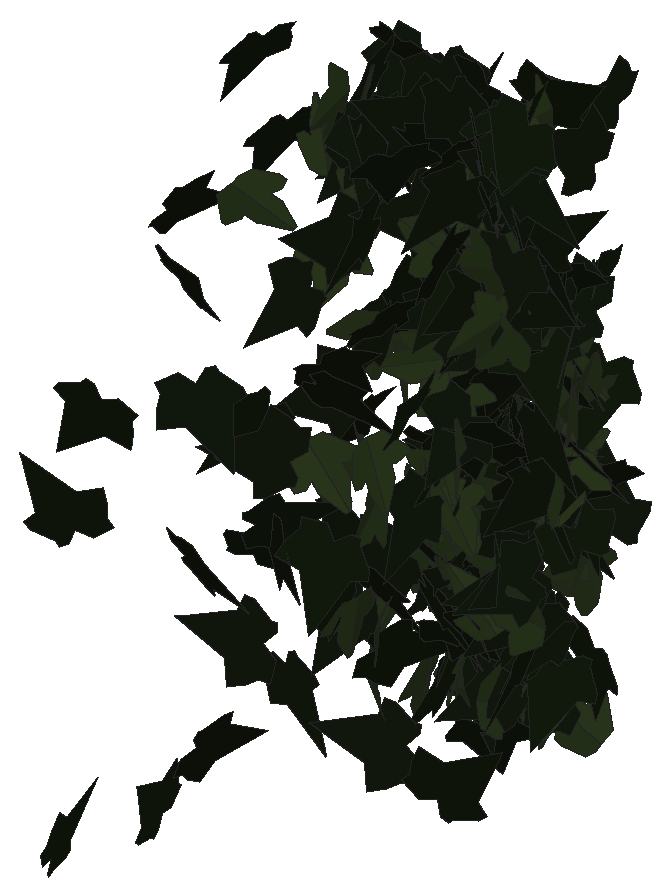
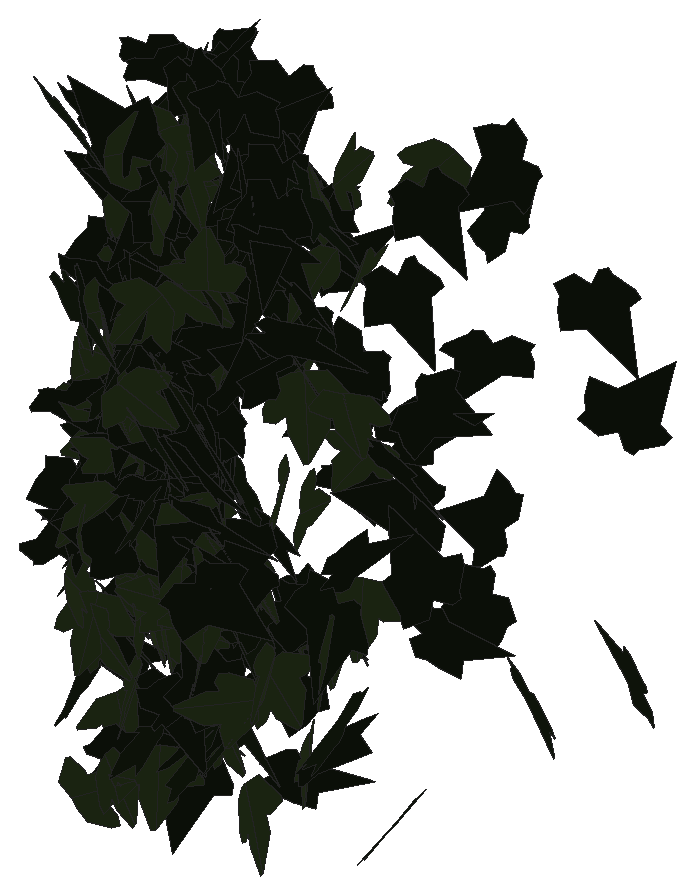
# SketchUp Ruby script. Lengths in inches.
U = 1.inch
M = Sketchup.active_model
def pt(a) = Geom::Point3d.new(a.map { |v| v * U })
def face(e, loops, mat)
  f = e.add_face(loops[0].map { |a| pt(a) })
  loops[1..].each { |l| e.add_face(l.map { |a| pt(a) }).erase! }
  f.material = f.back_material = mat if mat
  f
end
# faces: each face lists its corners as indices into pts; further lists are holes
def faces(e, pts, list, mat = nil) = list.each { |f| face(e, (f[0].is_a?(Array) ? f : [f]).map { |l| l.map { |i| pts[i] } }, mat) }
# xy, xz, yz: faces in a plane at the given z, y or x. An outline is a flat list of corners, or four numbers for a rectangle; further outlines are holes
def ring(l) = l.size == 4 ? [[l[0], l[1]], [l[2], l[1]], [l[2], l[3]], [l[0], l[3]]] : l.each_slice(2).to_a
def flat(e, list, mat, &to3) = list.each { |f| face(e, (f[0].is_a?(Array) ? f : [f]).map { |l| ring(l).map { |u, v| to3.(u, v) } }, mat) }
def xy(e, z, list, mat = nil) = flat(e, list, mat) { |x, y| [x, y, z] }
def xz(e, y, list, mat = nil) = flat(e, list, mat) { |x, z| [x, y, z] }
def yz(e, x, list, mat = nil) = flat(e, list, mat) { |y, z| [x, y, z] }
def lines(e, pts, list) = list.each { |a, b| e.add_line(pt(pts[a]), pt(pts[b])) }
# prism: a flat outline (further loops are holes) pulled along v
def prism(e, loops, v, mat = nil)
  f = face(e, loops, mat); d = Geom::Vector3d.new(v.map { |x| x * U })
  f.pushpull(f.normal.samedirection?(d) ? d.length : -d.length)
end
def box(e, o, s, mat = nil) = prism(e, [[o, [o[0] + s[0], o[1], o[2]], [o[0] + s[0], o[1] + s[1], o[2]], [o[0], o[1] + s[1], o[2]]]], [0, 0, s[2]], mat)
def at(x, y, z, deg = 0) = Geom::Transformation.translation(pt([x, y, z])) * Geom::Transformation.rotation(ORIGIN, Z_AXIS, deg.degrees)
def axes(o, x, y, z) = Geom::Transformation.new([*x, 0, *y, 0, *z, 0, *pt(o).to_a, 1])
def part(name) = M.definitions.add(name)
# library, detail: a bought-in or finely detailed component or shape, given as its bounding box
def library(name, o, s) = part(name).tap { |d| box(d.entities, o, s) }
def detail(e, o, s) = box(e.add_group.entities, o, s)
def put(e, d, t, mat = nil) = e.add_instance(d, t).tap { |i| i.material = mat if mat }
def group(e, t, mat = nil) = e.add_group.tap { |g| g.transformation = t; g.material = mat if mat }.entities
root = M.entities
M.materials.add("efeu1").color = [18, 25, 13]
M.materials.add("efeu2").color = [43, 57, 29]
c1 = part("ivyleaf_9")
p = [[1.54,2.16,1.25],[1.36,2.04,1.19],[-0.21,0.99,0.68],[-0.71,1.11,0.82],[-0.85,0.86,0.67],[-0.8,0.17,0.21],
  [-0.9,-0.01,0.1],[-0.67,-0.16,-0.02],[-0.08,-0.08,-0.05],[-0.03,-0.6,-0.4],[0.65,-0.88,-0.66],[0.83,-0.6,-0.49],
  [1.29,-0.42,-0.43],[1.8125,-0.07,-0.26],[1.21,0.44,0.15]]
faces(c1.entities,p,[[0,1,2,3,4,5,6,7,8,9,10,11,12,13,14]],"efeu1")
c2 = part("ivyleaf_10")
p = [[0,0.5,-0.03],[-0.0625,2.02,-0.43],[-0.19,2.01,-0.46],[-0.54,1.05,-0.29],[-0.52,0.625,-0.18],[-0.83,0.76,-0.28],
  [-1.16,0.64,-0.33],[-1.15,0.33,-0.24],[-0.77,-0.39,0.02],[-0.3,-0.51,0.16],[0.04,-0.48,0.23],[-0.02,2.01,-0.4375],
  [-0.06,2.01,-0.43],[0.04,-0.49,0.23],[0.67,-0.49,0.14],[1.38,0.36,-0.2],[1.375,0.51,-0.24],[0.81,0.65,-0.19],
  [0.62,0.59,-0.15],[0.6,1.09,-0.28],[0.5,1.23,-0.31]]
faces(c2.entities,p,[[0,1,2,3,4,5,6,7,8,9,10],[11,12,0,13,14,15,16,17,18,19,20]],"efeu2")
put(root,c1,axes([1.99,221.875,233.01],[-0.08667,0.34716,-0.25952],[0.03326,-0.24854,-0.3699],[-0.46054,-0.08328,0.02212]))
put(root,c1,axes([2.25,217.34,227.28],[0.20466,0.0164,0.40686],[-0.41836,0.07126,0.19203],[-0.06169,-0.42881,0.04747]))
put(root,c1,axes([2.25,222.11,231.66],[-0.04904,0.3605,-0.24874],[0.02338,-0.23829,-0.37781],[-0.46665,-0.04982,0.00721]))
put(root,c1,axes([2.48,222.28,229.01],[-0.46717,0.04349,-0.01539],[0.01585,-0.002,-0.45214],[-0.04701,-0.43282,0.00054]))
put(root,c1,axes([2.625,217.46,229.35],[0.16446,0.14018,-0.39791],[-0.29716,-0.26589,-0.21521],[-0.32459,0.31445,-0.00459]))
put(root,c2,axes([2.54,223.28,226.6],[-0.27724,0.37419,0.18198],[-0.15029,0.11386,-0.46309],[-0.38801,-0.31147,0.04934]))
put(root,c1,axes([2.81,222.76,227.24],[-0.16683,-0.15113,0.39263],[-0.24702,-0.30162,-0.2229],[0.36313,-0.27461,0.02875]))
put(root,c1,axes([2.79,222.78,226.72],[0.04672,0.47615,0.14526],[0.02368,0.14361,-0.47835],[-0.49725,0.05157,-0.00913]))
put(root,c1,axes([2.49,221.82,223.11],[0.22349,-0.37596,-0.07396],[-0.01378,0.07402,-0.44561],[0.41301,0.20591,0.02515]))
put(root,c1,axes([2.5,223,225.0625],[0.3031,-0.39745,-0.01273],[-0.00731,0.01043,-0.49984],[0.39759,0.30319,0.00051]))
put(root,c1,axes([2.71,216.32,222.62],[-0.16132,0.38355,0.14635],[0.04529,-0.13465,0.42797],[0.4389,0.15487,0.00963]))
put(root,c2,axes([2.93,222.1,226.56],[-0.45699,-0.09118,0.04487],[-0.04877,0.00485,-0.44993],[0.09742,-0.42531,-0.01475]))
put(root,c2,axes([2.8,222.51,229.72],[0.45214,0.11105,-0.0419],[-0.03967,-0.01863,-0.45037],[-0.12126,0.42017,-0.0089]))
put(root,c1,axes([2.77,218.87,231.89],[0.18453,0.28347,0.29356],[0.16249,0.23886,-0.3442],[-0.40032,0.22763,-0.00439]))
put(root,c2,axes([2.98,222.02,231.375],[-0.00592,0.38029,-0.21958],[-0.10567,0.20466,0.38602],[0.45772,0.05217,0.08628]))
put(root,c1,axes([3.22,223.65,231.15],[-0.45175,-0.09101,0.194],[-0.18219,-0.07516,-0.45952],[0.1128,-0.48587,0.03475]))
put(root,c1,axes([3.5625,219.87,224.75],[-0.24563,-0.1202,-0.36482],[-0.29899,-0.21873,0.26462],[-0.26643,0.35628,0.03937]))
put(root,c1,axes([3.48,217.76,222.94],[-0.15622,0.29714,0.29418],[-0.12907,0.2564,-0.34367],[-0.42385,-0.18759,-0.00377]))
put(root,c1,axes([2.9375,218.88,230.81],[0.41631,-0.10715,-0.17758],[0.18566,-0.01772,0.41517],[-0.11371,-0.42122,0.02771]))
put(root,c1,axes([3.2,222.55,224.21],[-0.1375,-0.42357,0.22735],[-0.07995,-0.21302,-0.44523],[0.47403,-0.15879,-0.00915]))
put(root,c1,axes([3.07,219.08,229.03],[-0.11466,-0.27255,-0.33486],[0.13265,0.29766,-0.30417],[0.43585,-0.16229,0.00448]))
put(root,c1,axes([3.04,220.4375,225.78],[0.42927,0.17672,0.00344],[-0.00574,0.00381,0.45235],[0.19081,-0.39747,0.00587]))
put(root,c1,axes([2.9375,219.05,226.26],[0.28554,-0.20433,0.28966],[0.23374,-0.17538,-0.34747],[0.29077,0.34164,-0.00513]))
put(root,c1,axes([3.48,223.19,232.88],[0.3501,0.18259,-0.30675],[-0.31184,-0.05269,-0.38727],[-0.17375,0.46248,0.07698]))
put(root,c1,axes([3.49,223.52,232.5],[-0.4638,-0.157,-0.10121],[0.09193,0.04399,-0.4895],[0.1626,-0.47267,-0.01194]))
put(root,c1,axes([3.56,222.57,232.8125],[-0.38655,0.23158,-0.21668],[0.15656,-0.15774,-0.44789],[-0.2758,-0.41411,0.04944]))
put(root,c1,axes([3.54,220.03,228.41],[-0.07763,0.05244,-0.44284],[0.10395,-0.41876,-0.07054],[-0.45153,-0.10542,0.05989]))
put(root,c2,axes([3.45,221.78,232.63],[0.00638,0.00374,0.45234],[0.19753,-0.39468,0.00095],[0.42621,0.18286,-0.00721]))
put(root,c2,axes([3.4,219.73,232.01],[-0.27728,-0.16504,-0.32235],[0.30342,0.13379,-0.31612],[0.22751,-0.37959,0.02873]))
put(root,c2,axes([3.5,222.14,231.5],[0.01777,0.42576,0.26155],[0.01888,0.26096,-0.42608],[-0.49933,0.02502,-0.0068]))
put(root,c2,axes([3.57,223.29,225.75],[-0.29611,0.33767,-0.00558],[0.00783,-0.00102,-0.45234],[-0.36465,-0.27423,-0.00518]))
put(root,c1,axes([3.48,222.93,231.54],[-0.33559,-0.13983,-0.34325],[0.35765,-0.00063,-0.34941],[0.09729,-0.48005,0.10044]))
put(root,c1,axes([3.875,220.07,227.71],[-0.14385,-0.05873,0.42632],[-0.40868,-0.15765,-0.15136],[0.18167,-0.40115,-0.00293]))
put(root,c2,axes([3.57,222.04,232.1],[0.24086,-0.3692,0.05865],[-0.02925,0.04953,0.44857],[-0.4023,-0.22464,0.00251]))
put(root,c1,axes([3.79,222.23,231.98],[-0.45385,-0.11206,-0.00905],[0.00687,0.00992,-0.45223],[0.12119,-0.4202,-0.00827]))
put(root,c1,axes([3.57,219.87,226.67],[0.14422,0.29854,-0.2983],[0.08404,0.27791,0.3385],[0.43915,-0.15122,0.03319]))
put(root,c2,axes([3.77,222.71,228.28],[-0.21571,0.37048,-0.11432],[0.03937,-0.10512,-0.43735],[-0.41549,-0.2023,0.0179]))
put(root,c1,axes([4.12,221.25,230.75],[-0.07581,-0.07614,0.43939],[-0.3249,-0.29669,-0.10759],[0.33077,-0.30887,-0.00497]))
put(root,c2,axes([4.09,221.85,229.2],[-0.36431,-0.3403,0.03838],[-0.02642,-0.02794,-0.49852],[0.34144,-0.36526,0.00238]))
put(root,c2,axes([4.21,221.61,223.59],[-0.20681,0.15234,0.37403],[-0.28851,0.24113,-0.25415],[-0.30774,-0.32844,-0.0131]))
put(root,c1,axes([4.32,220.78,225.27],[-0.29273,0.11583,-0.33271],[-0.3246,0.11018,0.30632],[0.17221,0.40456,0.01183]))
put(root,c2,axes([4.04,222.56,225.05],[-0.10879,-0.41516,0.25653],[0.07131,-0.27353,-0.41242],[0.48278,-0.05315,0.11873]))
put(root,c1,axes([3.94,222.06,232.14],[-0.08696,-0.49197,0.02003],[-0.0023,-0.01993,-0.4996],[0.49237,-0.08698,0.0012]))
put(root,c1,axes([3.76,219.95,226.52],[0.07131,-0.07178,-0.44088],[0.46114,-0.03943,0.07611],[-0.05454,-0.42722,0.06705]))
put(root,c1,axes([3.94,221.59,231.86],[-0.26895,0.12998,0.34542],[0.29291,-0.19406,0.29047],[0.25016,0.36697,0.03126]))
put(root,c2,axes([4.15,222.9,223.29],[0.10572,-0.48775,-0.0303],[-0.00248,0.03046,-0.49906],[0.48869,0.10568,0.00402]))
put(root,c1,axes([4.49,221.76,225.72],[-0.0606,-0.01815,-0.44822],[-0.34295,-0.29242,0.0558],[-0.31531,0.32154,0.02545]))
put(root,c1,axes([4.01,223.09,232.08],[-0.00977,0.08005,0.44458],[0.09557,-0.41829,0.08341],[0.45987,0.08863,-0.00789]))
put(root,c1,axes([4.17,217.77,224.21],[-0.06467,0.18591,-0.40423],[-0.11356,0.37425,0.20302],[0.45126,0.12082,-0.00684]))
put(root,c1,axes([4.17,220.53,229.15],[0.29596,0.33081,0.07125],[0.03683,0.06067,-0.44657],[-0.363,0.27587,0.01278]))
put(root,c1,axes([4.39,221.6,229.41],[-0.4195,0.13152,-0.15091],[0.14442,-0.05736,-0.42634],[-0.15453,-0.41065,0.01122]))
put(root,c1,axes([4.34,222,232.62],[0.32376,0.20276,-0.251],[-0.21936,-0.13045,-0.37635],[-0.26034,0.36207,0.00496]))
put(root,c2,axes([4.0625,220.46,227.68],[0.30921,0.21533,0.25663],[0.21546,0.14525,-0.37255],[-0.2805,0.34894,-0.00328]))
put(root,c1,axes([4.31,222.23,231.375],[0.37407,-0.00943,-0.27352],[-0.28063,0.05665,-0.358],[0.04505,0.43119,0.04105]))
put(root,c2,axes([4.09,223.21,224.98],[-0.01672,0.00327,-0.4521],[0.35425,0.28556,-0.00991],[0.30813,-0.32813,-0.01313]))
put(root,c1,axes([4.08,220.6,228.73],[0.45298,0.06085,0.10193],[0.1049,0.01318,-0.44077],[-0.06724,0.43052,-0.00092]))
put(root,c2,axes([4.39,220.97,225.14],[-0.03365,-0.43265,-0.03396],[0.00769,0.03223,-0.4511],[0.46853,-0.0316,0.00497]))
put(root,c1,axes([4.55,223.54,226.75],[-0.0085,0.10038,-0.44011],[-0.07126,-0.41863,-0.10199],[-0.46429,0.06241,0.02371]))
put(root,c1,axes([4.18,223.26,224.46],[0.22834,-0.37929,-0.02689],[-0.01346,0.02265,-0.4516],[0.41036,0.21179,0.00015]))
put(root,c2,axes([4.61,222.45,226.66],[0.32005,-0.15546,-0.28903],[-0.25866,0.1414,-0.34785],[0.22666,0.38087,0.01117]))
put(root,c1,axes([4.43,223.4,228.83],[-0.35811,0.00864,-0.29269],[0.29989,-0.06197,-0.34222],[-0.05036,-0.43048,0.0434]))
put(root,c1,axes([4.36,222.16,229.53],[0.01565,-0.00408,0.45213],[0.32458,0.31441,-0.00735],[-0.33928,0.30059,0.01383]))
put(root,c1,axes([4.83,221.47,222.85],[-0.20929,-0.21605,-0.33699],[-0.2366,-0.23876,0.30183],[-0.34775,0.29248,-0.00254]))
put(root,c1,axes([4.15,222.71,226.88],[0.4228,-0.03831,0.19318],[0.19984,-0.01638,-0.40908],[0.04496,0.433,0.00162]))
put(root,c1,axes([4.59,222.63,229.33],[-0.20526,-0.27618,0.28826],[0.17014,0.22806,0.34867],[-0.38682,0.24686,0.00039]))
put(root,c1,axes([4.41,221.24,225.53],[0.46646,-0.00958,-0.05295],[-0.05492,0.00338,-0.44928],[0.01071,0.43488,0.00232]))
put(root,c2,axes([4.79,222.02,226.14],[-0.1037,0.34792,-0.25253],[-0.05961,0.2366,0.37527],[0.45432,0.11046,-0.0084]))
put(root,c1,axes([4.74,220.98,229.82],[0.16126,0.38704,0.13611],[0.02316,0.13173,-0.43058],[-0.44065,0.14856,0.02718]))
put(root,c1,axes([4.56,221.29,224.36],[0.03814,0.19653,-0.40192],[0.0246,0.38637,0.2065],[0.4676,-0.03636,0.02192]))
put(root,c2,axes([4.68,221.125,226.83],[-0.00437,0.15271,-0.42359],[0.00172,-0.4073,-0.15884],[-0.46978,-0.00291,0.00336]))
put(root,c1,axes([4.9,221.84,232.63],[0.00738,-0.00538,0.45231],[-0.38699,-0.24662,0.00268],[0.26626,-0.3583,-0.00863]))
put(root,c1,axes([4.86,220.74,231.58],[-0.38076,0.17298,-0.19459],[0.17299,-0.09797,-0.40809],[-0.21403,-0.38692,0.01633]))
put(root,c1,axes([4.5625,223.125,224.82],[0.25779,0.33704,0.14203],[-0.08328,-0.11274,0.42952],[0.38382,-0.25084,-0.0022]))
put(root,c2,axes([4.69,223.22,226.18],[0.30572,0.32986,0.01756],[0.01274,0.01213,-0.45206],[-0.35649,0.28332,-0.0011]))
put(root,c2,axes([4.65,221.26,224.89],[-0.01474,-0.13913,-0.4284],[0.1292,-0.39742,0.13548],[-0.45145,-0.10919,0.05276]))
put(root,c1,axes([5.17,222.3,226.7],[-0.22659,0.28825,0.2592],[-0.15637,0.20287,-0.37078],[-0.38068,-0.25491,-0.00198]))
put(root,c1,axes([5.12,221.96,231.19],[-0.16645,-0.09187,0.41212],[-0.38425,-0.17498,-0.18611],[0.21297,-0.38751,-0.01367]))
put(root,c1,axes([4.85,219.89,226.77],[-0.33375,-0.27698,-0.13562],[0.11742,0.07391,-0.43124],[0.30908,-0.32717,0.01739]))
put(root,c2,axes([5.02,223.04,224.93],[0.04987,-0.02167,-0.44928],[-0.13014,0.41661,-0.03513],[0.44865,0.12325,0.03975]))
put(root,c1,axes([5.27,222.83,227.22],[-0.34123,0.10886,0.28961],[-0.29696,0.05334,-0.34614],[-0.12683,-0.41777,0.03128]))
put(root,c2,axes([4.9375,223.08,226.82],[0.3059,-0.30462,-0.13239],[-0.04478,0.13358,-0.42838],[0.35374,0.28033,0.06026]))
put(root,c1,axes([5.28,223.37,224.47],[-0.17419,-0.01615,0.41982],[-0.43468,-0.03122,-0.16854],[0.03779,-0.43358,-0.00351]))
put(root,c1,axes([5.3,222.81,228.02],[-0.21573,0.21724,0.33237],[-0.26457,0.20704,-0.3056],[-0.32276,-0.31491,0.02836]))
put(root,c2,axes([5.15,222.875,225.9375],[-0.42482,0.0594,-0.18303],[-0.18604,0.03747,0.41358],[0.07502,0.42929,-0.01077]))
put(root,c1,axes([4.69,222.06,225.77],[0.44786,-0.12359,0.04635],[0.05602,0.01845,-0.44876],[0.13037,0.41666,0.03362]))
put(root,c1,axes([5.24,221.75,225.39],[-0.06242,0.37466,0.22187],[-0.12707,0.19337,-0.38633],[-0.44796,-0.10706,0.07867]))
put(root,c2,axes([5.31,221.6,229.14],[0.19377,0.01768,-0.41171],[-0.42779,0.02095,-0.18573],[0.01276,0.43414,0.02573]))
put(root,c1,axes([5.09,221.62,226.8],[-0.43427,-0.01849,-0.1715],[0.17778,0.0102,-0.41862],[0.02265,-0.43449,-0.00253]))
put(root,c2,axes([5.35,222.125,223.73],[-0.12751,0.0389,0.43354],[-0.43058,0.12178,-0.12925],[-0.13804,-0.41579,0.00271]))
put(root,c2,axes([4.9375,221.9375,226.22],[-0.36008,0.21677,-0.18332],[0.14584,-0.11524,-0.41301],[-0.26417,-0.3591,0.02188]))
put(root,c1,axes([5.28,222.9375,226.82],[-0.46754,0.00477,0.04405],[-0.04601,-0.0324,-0.44896],[-0.0017,-0.43377,0.03402]))
put(root,c1,axes([4.92,221.5,232.68],[0.44215,0.14489,-0.02596],[-0.02427,-0.01133,-0.45164],[-0.15692,0.41001,-0.00331]))
put(root,c1,axes([4.98,222.41,227.37],[0.0093,0.07598,0.44535],[-0.05382,-0.42532,0.07953],[0.46661,-0.05057,0.00029]))
put(root,c1,axes([5.35,223.15,224.8],[0.16925,0.14218,-0.39527],[-0.35904,-0.18865,-0.21596],[-0.25131,0.36527,0.04232]))
put(root,c1,axes([5.3125,221.93,223.96],[-0.36308,0.24318,-0.13586],[0.10904,-0.08328,-0.43144],[-0.27747,-0.35093,0.00824]))
put(root,c1,axes([5.39,222.33,229.92],[-0.04027,-0.03124,-0.44956],[-0.15044,-0.40998,0.04331],[-0.44323,0.14199,0.02615]))
put(root,c1,axes([4.99,222.16,233.5],[-0.15779,-0.23335,-0.35026],[0.18037,0.29259,-0.28619],[0.40408,-0.22173,-0.00903]))
put(root,c2,axes([5.05,223.04,225.34],[-0.29761,0.28093,-0.1928],[0.13782,-0.1345,-0.40925],[-0.33637,-0.30367,0.00291]))
put(root,c2,axes([5.27,222.82,227.37],[0.37561,0.18131,-0.19567],[-0.191,-0.06723,-0.40737],[-0.20773,0.38966,0.02076]))
put(root,c1,axes([5.32,221.58,227.24],[-0.27821,0.31054,-0.16908],[-0.14463,0.09926,0.41787],[0.34984,0.28799,0.0383]))
put(root,c1,axes([5,222.55,229.02],[-0.1911,-0.05911,-0.40868],[0.39998,0.13143,-0.19399],[0.1556,-0.41044,-0.00326]))
put(root,c2,axes([5.2,222.53,230.82],[0.39875,0.22919,-0.02016],[0.01508,0.01425,0.45192],[0.24795,-0.36945,0.00492]))
put(root,c2,axes([5.29,221.63,230.91],[-0.12516,0.33022,0.26869],[0.01756,-0.2643,0.35892],[0.45248,0.1016,0.06039]))
put(root,c2,axes([5.64,222.83,225.45],[0.02935,0.02469,0.45079],[-0.44534,-0.13441,0.03485],[0.1467,-0.41298,0.01561]))
put(root,c1,axes([5.47,221.74,228.58],[0.17857,-0.0339,-0.41696],[-0.42842,0.05877,-0.17531],[0.07269,0.42968,-0.00892]))
put(root,c2,axes([5.23,222.03,226.64],[0.05136,0.40773,0.14971],[0.02268,0.14247,-0.42689],[-0.46643,0.05183,-0.00427]))
put(root,c1,axes([5.02,223.01,223.68],[0.29387,-0.32324,0.10758],[0.08252,-0.07084,-0.43923],[0.35713,0.28235,0.01297]))
put(root,c1,axes([5.44,220.5,232.91],[0.12181,0.39904,-0.13668],[-0.05723,-0.12147,-0.43089],[-0.45011,0.12344,0.01779]))
put(root,c2,axes([5.35,222.16,224.23],[0.29022,-0.34153,-0.02006],[-0.01195,0.01583,-0.45195],[0.36924,0.26895,0.00114]))
put(root,c1,axes([5.18,222.74,223.76],[0.00195,-0.42695,-0.0866],[0.02606,0.08324,-0.44333],[0.46907,-0.00285,0.02499]))
put(root,c1,axes([5.65,222.69,229.07],[-0.15183,0.28905,0.30483],[-0.17894,0.2438,-0.33269],[-0.40699,-0.21503,0.03255]))
put(root,c1,axes([5.53,222.17,233.11],[-0.00466,0.30865,0.31875],[-0.04788,0.3046,-0.31967],[-0.46733,-0.03429,0.02957]))
put(root,c1,axes([5.2,222.39,227.81],[-0.05974,0.11809,0.43159],[0.10786,-0.40352,0.13326],[0.45333,0.11157,0.02516]))
put(root,c1,axes([5.05,222.51,228.05],[0.20991,0.03915,0.40268],[0.411,0.07139,-0.20618],[-0.08789,0.42731,-0.00245]))
put(root,c1,axes([5.43,222.68,227.48],[0.37776,0.20394,-0.16537],[-0.16377,-0.05491,-0.42016],[-0.22624,0.38029,0.02802]))
put(root,c2,axes([5.69,222.6,230.57],[-0.16371,-0.19818,0.37058],[-0.24512,-0.2748,-0.25937],[0.36582,-0.27282,-0.00795]))
put(root,c1,axes([5.57,221.72,225.13],[0.29817,0.08409,-0.33849],[-0.34193,-0.07654,-0.29986],[-0.12205,0.41988,0.01313]))
put(root,c1,axes([5.26,221.57,225.41],[0.39031,-0.22645,-0.08907],[-0.07396,0.052,-0.44347],[0.25079,0.36775,0.00785]))
put(root,c2,axes([5.54,222.54,227.3],[-0.41656,-0.2008,-0.01201],[0.01282,0.00222,-0.45223],[0.21685,-0.38587,0.00365]))
put(root,c2,axes([5.64,223.06,223.44],[-0.39943,-0.22884,0.00901],[-0.00792,-0.00462,-0.45231],[0.2472,-0.36991,0.00007]))
put(root,c2,axes([5.7,223.6,229.39],[0.2407,0.23237,-0.3042],[-0.26017,-0.17093,-0.33211],[-0.30836,0.32559,0.04276]))
put(root,c1,axes([5.86,221.93,230.59],[-0.10752,0.34488,0.25553],[-0.16195,0.20733,-0.36585],[-0.4277,-0.16521,0.0743]))
put(root,c1,axes([5.34,221.9,231.07],[0.40358,-0.22265,-0.00362],[0.00765,0.01869,-0.45192],[0.24037,0.37323,0.02047]))
put(root,c2,axes([5.51,222.95,225.92],[-0.02374,-0.22179,0.38851],[0.07223,0.36786,0.23123],[-0.46361,0.06867,0.01613]))
put(root,c1,axes([5.52,221.59,225.01],[0.37577,0.25902,0.03412],[0.02457,0.02439,-0.45107],[-0.2809,0.34862,0.0062]))
put(root,c1,axes([5.89,222.02,233.56],[0.13365,0.10043,-0.42094],[-0.4252,-0.11107,-0.15385],[-0.1485,0.40841,0.06167]))
put(root,c1,axes([5.69,222.23,223.13],[0.28755,0.32531,-0.11632],[-0.08111,-0.08305,-0.43716],[-0.36255,0.27659,0.00554]))
put(root,c1,axes([5.8,221.77,230.54],[-0.4122,-0.2084,0.01143],[-0.01056,-0.00504,-0.45226],[0.22514,-0.38179,-0.00027]))
put(root,c2,axes([5.62,219.8125,228.54],[0.06028,0.42821,0.0545],[0.00897,0.05176,-0.4491],[-0.46583,0.05641,-0.00159]))
put(root,c1,axes([5.47,223.29,224.2],[0.40234,-0.28702,-0.07581],[-0.05613,0.05182,-0.49413],[0.2915,0.40612,0.00948]))
put(root,c1,axes([5.79,222,227.65],[0.04979,0.24521,0.37059],[0.04959,0.35355,-0.2592],[-0.46452,0.06402,0.01205]))
put(root,c1,axes([5.9,223.21,228.85],[-0.39551,0.20609,-0.11691],[0.1025,-0.06054,-0.43699],[-0.23189,-0.37827,0.00624]))
put(root,c2,axes([5.94,222.22,232.17],[-0.39995,-0.07157,0.22537],[-0.22671,-0.05523,-0.39205],[0.0967,-0.4255,0.01298]))
put(root,c1,axes([6.04,222.97,227.34],[-0.31722,-0.28143,-0.16028],[-0.12069,-0.10612,0.42306],[-0.32484,0.31426,-0.00067]))
put(root,c2,axes([5.8,222.69,225.54],[0.20348,-0.44688,-0.09431],[-0.02633,0.0916,-0.49083],[0.45596,0.20472,0.01374]))
put(root,c1,axes([5.59,221.93,228.05],[0.07695,0.42436,-0.06631],[0.01058,0.06301,0.44751],[0.46333,-0.07192,0.0008]))
put(root,c2,axes([5.88,222.11,223.63],[-0.04663,0.14675,0.42351],[-0.12251,0.3911,-0.15909],[-0.45114,-0.12137,-0.00057]))
put(root,c1,axes([6.13,222.33,223.94],[-0.45302,0.03049,0.11557],[-0.1208,-0.00681,-0.43713],[-0.02994,-0.43388,0.01498]))
put(root,c1,axes([5.98,221.62,229.98],[-0.33018,0.24358,-0.19849],[0.15615,-0.12477,-0.40647],[-0.29548,-0.33812,0.007]))
put(root,c2,axes([5.77,223.32,225.77],[-0.07556,0.09542,-0.43534],[0.04075,-0.42111,-0.10639],[-0.46189,-0.05276,0.06183]))
put(root,c2,axes([5.57,223.05,231.73],[-0.09606,-0.07468,0.43598],[0.41888,-0.19096,0.05021],[0.1898,0.38364,0.10985]))
put(root,c1,axes([5.97,220.77,231.23],[-0.12236,0.21356,-0.3761],[-0.25468,0.2776,0.24732],[0.37534,0.25799,0.04521]))
put(root,c1,axes([5.69,222.8,227.54],[-0.04359,0.17142,0.41367],[0.08802,-0.38934,0.18311],[0.45942,0.09086,0.00417]))
put(root,c1,axes([5.68,223.16,227.48],[0.32742,-0.28663,-0.12803],[-0.098,0.08321,-0.4339],[0.32234,0.31645,-0.00187]))
put(root,c1,axes([5.63,222.04,229.49],[0.17907,-0.30508,-0.35336],[0.02402,0.38398,-0.31934],[0.46622,0.09739,0.15218]))
put(root,c2,axes([5.97,222.44,231.94],[-0.04732,0.39382,-0.18666],[-0.01913,0.17862,0.41209],[0.46702,0.04722,-0.00203]))
put(root,c2,axes([5.76,221.375,228.95],[0.40178,0.19262,0.12184],[0.09159,0.08988,-0.43376],[-0.2256,0.37953,0.04089]))
put(root,c2,axes([5.93,222.88,225.67],[0.21874,-0.38138,0.05456],[0.02891,-0.04518,-0.44909],[0.41477,0.20428,0.00254]))
put(root,c1,axes([5.81,222.69,232.29],[-0.06841,0.34286,0.27053],[0.05456,-0.25518,0.36259],[0.46158,0.08098,-0.00277]))
put(root,c1,axes([6.07,222.87,229.6875],[-0.42707,-0.17817,-0.0347],[0.03312,0.01315,-0.45107],[0.19294,-0.39662,0.00063]))
put(root,c2,axes([5.89,222.8125,229.02],[-0.05062,0.3956,-0.18172],[0.02699,-0.17298,-0.41428],[-0.46628,-0.05296,-0.00425]))
put(root,c2,axes([5.96,222.52,232.68],[0.31439,0.30369,-0.11513],[-0.08965,-0.07375,-0.43741],[-0.33739,0.30258,0.00895]))
put(root,c2,axes([5.82,223.01,230.42],[-0.39031,0.02946,-0.24992],[0.25696,-0.03667,-0.3768],[-0.04838,-0.43245,0.01493]))
put(root,c1,axes([5.78,221.41,233.62],[0.18877,-0.44629,-0.12324],[-0.03279,0.11987,-0.48431],[0.46183,0.19093,0.01599]))
put(root,c2,axes([6.23,221.65,225.29],[0.33097,0.1086,0.30056],[-0.29039,-0.10623,0.33803],[0.16385,-0.40761,-0.00802]))
put(root,c1,axes([6.31,223.3,223.37],[-0.25905,-0.26739,-0.25517],[-0.06865,-0.2586,0.35772],[-0.38587,0.22551,0.10766]))
put(root,c2,axes([6.35,222.96,226.03],[0.14044,0.00832,0.43163],[-0.44544,0.05176,0.13332],[-0.05069,-0.43183,0.02429]))
put(root,c1,axes([6.02,220.94,232.87],[0.19164,0.33213,0.22649],[0.09009,0.20204,-0.39114],[-0.41937,0.19518,0.01948]))
put(root,c2,axes([6.09,223.31,232.76],[0.01374,-0.05639,0.44839],[0.01934,-0.43089,-0.05916],[0.4692,0.01941,-0.01069]))
put(root,c2,axes([6.06,223.04,224.59],[-0.26917,0.355,0.03421],[-0.01503,0.03042,-0.45106],[-0.38475,-0.24955,-0.00632]))
put(root,c1,axes([5.95,222.47,231.83],[0.03798,-0.17915,-0.41063],[-0.06338,0.39052,-0.18971],[0.46395,0.06801,0.0077]))
put(root,c2,axes([6.125,223.42,223.32],[0.01163,-0.41504,0.13501],[0.00823,-0.12965,-0.43177],[0.46958,0.01255,0.00422]))
put(root,c1,axes([6.15,222.11,226.31],[-0.36689,0.26641,0.05552],[0.03868,-0.04082,0.44886],[0.29088,0.34145,0.01034]))
put(root,c1,axes([6.03,222.37,231.04],[0.44807,0.08362,-0.10455],[-0.1214,0.05722,-0.43296],[-0.07215,0.42303,0.07923]))
put(root,c2,axes([5.99,222.29,231.83],[0.0013,0.00868,-0.45231],[0.1164,-0.42136,-0.00844],[-0.45515,-0.10774,-0.00345]))
put(root,c1,axes([5.98,222.49,231.77],[0.04225,0.39985,-0.17344],[0.01146,0.16652,0.4178],[0.46776,-0.0402,0.00543]))
put(root,c1,axes([6.39,219.68,229.46],[-0.11062,0.36781,0.21677],[-0.06367,0.19994,-0.39707],[-0.45213,-0.11815,0.00288]))
put(root,c1,axes([6.36,222.92,229.19],[-0.01858,-0.15772,-0.42124],[-0.06474,-0.40062,0.16488],[-0.46495,0.06209,-0.00612]))
put(root,c2,axes([5.95,222.2,232.63],[0.37528,0.0014,0.27216],[0.2826,-0.00875,-0.36129],[0.00448,0.43491,-0.00814]))
put(root,c2,axes([6.03,223.13,226.87],[0.42811,-0.00893,0.18609],[0.19348,0.02321,-0.41155],[-0.00154,0.43429,0.02583]))
put(root,c1,axes([6.19,222.77,230.21],[0.35869,-0.10037,-0.27288],[-0.26633,0.09044,-0.36061],[0.14532,0.41349,0.01264]))
put(root,c2,axes([6.58,223.33,225.3],[-0.16645,0.05189,0.4196],[-0.43871,0.00318,-0.16181],[-0.02323,-0.43188,0.04923]))
put(root,c1,axes([6.11,221.73,228.98],[0.31674,0.2687,0.18314],[-0.13776,-0.12146,0.41366],[0.31845,-0.3198,-0.00322]))
put(root,c2,axes([6.27,222.99,228.54],[0.44023,-0.14979,-0.02617],[-0.02418,0.01203,-0.45163],[0.16225,0.40822,0.0037]))
put(root,c1,axes([6.11,221.68,228.17],[0.46094,0.08266,-0.0161],[-0.01691,-0.00057,-0.45211],[-0.08924,0.42707,0.00251]))
put(root,c1,axes([6.55,221.37,230.75],[0.04247,0.07295,-0.44411],[-0.26324,-0.35076,-0.08566],[-0.3868,0.24673,0.00954]))
put(root,c2,axes([6.57,223.49,222.79],[0.24514,0.09471,0.37315],[-0.36387,-0.1237,0.25562],[0.16799,-0.40614,0.00916]))
put(root,c1,axes([6.61,222.49,224.8125],[-0.39546,0.22777,0.05945],[-0.05754,0.02256,-0.44838],[-0.24701,-0.36991,0.00927]))
put(root,c1,axes([6.01,223.2,232.8],[-0.01629,-0.09471,0.44127],[0.41765,-0.19689,-0.03141],[0.21451,0.37615,0.09466]))
put(root,c1,axes([6.56,222.22,225.71],[-0.0741,-0.17468,-0.40813],[-0.0737,-0.38793,0.19199],[-0.45803,0.09068,0.03514]))
put(root,c1,axes([6.01,223.1875,226.74],[0.16088,-0.03426,0.42355],[0.43942,0.05336,-0.15011],[-0.04168,0.43035,0.05233]))
put(root,c1,axes([6.68,221.97,232.2],[-0.20167,0.33443,0.21443],[-0.14389,0.16086,-0.39684],[-0.39917,-0.22695,0.03471]))
put(root,c2,axes([6.39,222.58,229.45],[-0.43056,-0.16364,-0.06159],[0.07432,-0.01229,-0.44652],[0.17263,-0.40286,0.03864]))
put(root,c1,axes([6.54,222.5,227.23],[-0.02417,0.4322,0.0457],[-0.01025,0.0435,-0.45002],[-0.46907,-0.02322,0.00748]))
put(root,c1,axes([6.54,221.875,229.4],[0.01986,0.37295,-0.23207],[-0.03677,-0.22142,-0.38779],[-0.46794,0.03323,0.02062]))
put(root,c1,axes([6.43,222.61,228.86],[0.36036,0.17851,-0.22312],[-0.21443,-0.08319,-0.39312],[-0.21184,0.38787,0.01837]))
put(root,c1,axes([6.62,222.76,227.74],[0.21436,0.20398,-0.34213],[-0.33173,-0.14197,-0.28429],[-0.25439,0.35702,0.08243]))
put(root,c2,axes([6.41,221.34,232.61],[-0.23692,0.37531,-0.01627],[0.00858,-0.01348,-0.45211],[-0.4056,-0.21951,-0.00005]))
put(root,c1,axes([6.69,222.14,225.45],[0.03265,0.06233,-0.44663],[-0.14566,-0.40782,-0.07143],[-0.44545,0.13792,-0.00937]))
put(root,c2,axes([6.51,223.33,225.62],[-0.28259,-0.32627,-0.1244],[0.07892,0.09472,-0.43495],[0.36692,-0.27166,-0.00225]))
put(root,c2,axes([6.52,222.8,223.96],[0.22037,0.37082,-0.10445],[-0.07852,-0.07439,-0.43928],[-0.40741,0.21491,0.02817]))
put(root,c1,axes([6.69,222.52,230.27],[0.10695,-0.05135,0.43727],[-0.11837,0.41398,0.07943],[-0.44188,-0.12332,0.08456]))
put(root,c2,axes([6.74,222.24,231.4],[-0.29634,-0.22707,0.25974],[-0.17522,-0.19353,-0.36836],[0.31968,-0.31656,0.03888]))
put(root,c1,axes([6.65,221.27,232.37],[0.04843,-0.33116,0.28961],[0.00886,0.28056,0.34562],[-0.46721,-0.02901,0.03657]))
put(root,c1,axes([6.65,220.58,232.9],[-0.02117,0.09159,-0.44179],[0.08592,-0.41729,-0.09739],[-0.46139,-0.08191,0.00213]))
put(root,c2,axes([6.39,223.24,227.29],[0.13928,0.27631,0.32265],[0.15051,0.27725,-0.31705],[-0.42268,0.18977,-0.00658]))
put(root,c1,axes([6.53,222.55,230.66],[-0.36019,-0.10494,-0.26916],[0.26107,0.09341,-0.36335],[0.15105,-0.41169,-0.01383]))
put(root,c1,axes([6.29,223.16,229.2],[0.2847,-0.30195,0.17575],[0.11401,-0.13214,-0.41681],[0.35589,0.28388,-0.00707]))
put(root,c2,axes([6.47,222.32,230.54],[-0.36368,-0.10516,-0.26469],[0.26655,0.06308,-0.36671],[0.13192,-0.41736,0.01127]))
put(root,c1,axes([6.41,221.95,227.5],[0.06734,0.29643,-0.32469],[0.06721,0.30594,0.31503],[0.46007,-0.08808,0.0015]))
put(root,c2,axes([6.875,222.26,227.47],[0.26148,-0.14233,-0.34547],[-0.27951,0.2108,-0.29011],[0.27243,0.35289,0.03395]))
put(root,c2,axes([6.44,222.96,227.8],[0.36473,0.15411,0.23584],[0.22564,0.08835,-0.38602],[-0.19177,0.39707,-0.00564]))
put(root,c2,axes([6.38,223,229.02],[0.244,0.09746,0.37307],[0.33408,0.18349,-0.25446],[-0.22263,0.38217,0.02703]))
put(root,c2,axes([7.03,220.66,231.64],[-0.18953,0.01926,0.41347],[-0.42406,0.06285,-0.18342],[-0.07046,-0.43001,-0.00829]))
put(root,c2,axes([6.65,223.58,226.1],[0.14215,-0.29865,0.2991],[0.12463,-0.26343,-0.33942],[0.43009,0.17504,-0.0005]))
put(root,c1,axes([6.9,222.27,227.49],[0.02013,0.1056,-0.43844],[-0.10105,-0.41109,-0.1114],[-0.45836,0.09527,0.0053]))
put(root,c1,axes([6.45,222.94,227.64],[0.4649,-0.03034,0.05703],[0.05916,-0.00288,-0.44879],[0.03289,0.43393,0.00101]))
put(root,c1,axes([6.34,222.73,227.99],[0.3073,-0.23738,0.31499],[0.26719,-0.16844,-0.3876],[0.29013,0.40654,0.02333]))
put(root,c1,axes([6.81,221.9375,226.16],[-0.16756,-0.24541,0.33688],[-0.17645,-0.27981,-0.30185],[0.40187,-0.22518,0.00793]))
put(root,c1,axes([6.78,221.66,233.27],[-0.30184,-0.33331,0.00502],[-0.00158,-0.00508,-0.45237],[0.36,-0.27948,0.00223]))
put(root,c2,axes([6.58,221.66,231.27],[-0.20143,0.15918,-0.37368],[0.20832,-0.30944,-0.2467],[-0.36979,-0.26103,0.06457]))
put(root,c2,axes([6.58,223.46,226.84],[0.04464,-0.07819,0.44295],[0.28129,-0.33732,-0.09069],[0.37362,0.2633,0.01536]))
put(root,c1,axes([6.8125,222.32,230.73],[0.25756,0.34604,-0.11677],[-0.07477,-0.08863,-0.43702],[-0.38573,0.24824,0.00675]))
put(root,c2,axes([6.72,222.59,229.13],[-0.09352,0.40822,-0.12774],[0.01509,-0.12255,-0.43383],[-0.46015,-0.08698,0.01173]))
put(root,c1,axes([6.67,222.76,226.68],[0.32628,-0.20432,-0.24657],[-0.16597,0.19022,-0.37415],[0.29446,0.33361,0.06232]))
put(root,c1,axes([6.59,223.22,226.76],[0.14394,-0.40231,0.10192],[0.04783,-0.08851,-0.44053],[0.44464,0.13976,0.01439]))
put(root,c1,axes([6.97,222.34,225.17],[-0.44644,0.06421,-0.12405],[0.11317,-0.09121,-0.42871],[-0.09272,-0.42046,0.07405]))
put(root,c1,axes([6.6875,222.125,229.76],[-0.09545,-0.37465,-0.21071],[0.08205,0.18973,-0.39936],[0.45262,-0.1134,0.02796]))
put(root,c1,axes([6.92,221.63,233.42],[-0.40284,-0.21648,-0.05912],[0.04562,0.0404,-0.4483],[0.23738,-0.37514,-0.01416]))
put(root,c2,axes([6.87,222.97,229.94],[0.00388,0.12912,-0.43199],[-0.11736,-0.40196,-0.13092],[-0.45489,0.10481,0.0301]))
put(root,c1,axes([7.07,223.22,230.34],[-0.34888,0.28951,-0.03386],[0.02379,-0.02421,-0.45112],[-0.31374,-0.32377,0.00345]))
put(root,c1,axes([6.89,220.23,229.125],[0.25106,0.34963,-0.11834],[-0.07248,-0.09202,-0.43662],[-0.39042,0.24191,0.00495]))
put(root,c1,axes([6.84,220.46,229.26],[-0.17293,-0.36468,0.18191],[-0.0728,-0.16143,-0.4142],[0.43071,-0.17371,0.00303]))
put(root,c1,axes([6.91,221.69,224.96],[-0.32834,0.13168,-0.29315],[0.24378,-0.17788,-0.33961],[-0.23125,-0.37449,0.05823]))
put(root,c1,axes([7.24,222.71,230.15],[-0.30818,0.10559,0.32332],[-0.32093,0.09211,-0.3162],[-0.1508,-0.41181,0.01218]))
put(root,c2,axes([6.89,222.67,229.75],[0.30303,-0.3955,-0.04186],[-0.00803,0.04652,-0.49777],[0.39763,0.30235,0.02184]))
put(root,c1,axes([7.19,223.3,233.17],[-0.28101,0.29775,0.18855],[-0.14513,0.12307,-0.41079],[-0.34739,-0.29227,0.0191]))
put(root,c1,axes([6.67,221.84,232.4],[0.05854,-0.35966,0.24814],[0.06622,-0.23162,-0.37759],[0.46141,0.07887,0.02271]))
put(root,c1,axes([7.18,221.37,226.4],[-0.44872,0.06655,0.11474],[-0.11768,0.01729,-0.43761],[-0.07427,-0.42953,0.00016]))
put(root,c2,axes([7.25,221.28,225.76],[-0.04756,0.02899,-0.44906],[-0.45818,0.08284,0.05078],[0.09232,0.42605,0.02068]))
put(root,c1,axes([7.13,222.59,226.37],[-0.42978,-0.17007,0.04581],[0.04672,0.01087,0.45002],[-0.1839,0.40023,0.00725]))
put(root,c2,axes([7.1875,220.87,230.54],[-0.36618,-0.01801,0.2828],[-0.28793,-0.06806,-0.3504],[0.06102,-0.42926,0.04369]))
put(root,c1,axes([6.79,222.04,228.58],[0.25551,-0.30773,-0.20422],[-0.13386,0.15238,-0.40365],[0.37082,0.26704,-0.005]))
put(root,c1,axes([6.68,222.04,231.43],[0.34658,-0.35987,-0.0194],[-0.01992,0.00774,-0.49954],[0.35984,0.34704,-0.00897]))
put(root,c1,axes([7.03,222.96,227.28],[0.14399,0.40677,-0.08046],[-0.0383,-0.06977,-0.44502],[-0.44555,0.13746,0.01225]))
put(root,c1,axes([6.96,222.41,224.5],[-0.34948,-0.27747,-0.09023],[0.07906,0.04788,-0.44316],[0.30386,-0.33158,0.01152]))
put(root,c1,axes([6.84,223.21,230.3],[-0.20813,0.04125,-0.40331],[0.38724,-0.1514,-0.20205],[-0.16566,-0.40571,0.0344]))
put(root,c1,axes([6.93,223.37,228.84],[-0.2726,-0.34895,-0.06368],[0.04141,0.04783,-0.44789],[0.38038,-0.25528,0.00312]))
put(root,c1,axes([6.74,221.6,232.66],[0.30505,-0.31019,-0.24643],[-0.07223,0.26226,-0.41953],[0.38952,0.29155,0.11519]))
put(root,c2,axes([6.73,220.14,229.03],[0.34882,-0.13234,0.26999],[0.25896,-0.09952,-0.363],[0.17883,0.40225,-0.00098]))
put(root,c1,axes([7.33,222.58,232.61],[-0.22947,0.20464,0.33248],[-0.25476,0.21585,-0.30674],[-0.32117,-0.31743,0.00576]))
put(root,c1,axes([6.71,219.97,223.34],[-0.11416,-0.01516,0.43856],[0.43781,-0.12431,0.10103],[0.12649,0.41658,0.04611]))
put(root,c1,axes([6.77,223.33,224.24],[0.07516,-0.35381,0.25304],[0.05325,-0.23826,-0.37501],[0.46068,0.08527,0.00207]))
put(root,c1,axes([6.7,221.93,231.24],[0.0072,-0.01742,0.45198],[0.46663,0.05022,-0.0048],[-0.05399,0.43174,0.0188]))
put(root,c1,axes([7.1,223.32,226.3],[-0.34744,-0.20741,0.21494],[0.18528,0.11531,0.39806],[-0.25627,0.36457,-0.00362]))
put(root,c1,axes([6.97,221.25,231.54],[-0.35013,-0.23692,-0.174],[0.14572,0.09894,-0.4176],[0.27728,-0.35115,-0.00026]))
put(root,c1,axes([6.84,221.31,230.85],[0.09328,-0.03537,-0.44186],[-0.02997,0.43211,-0.04328],[0.45947,0.03537,0.08688]))
put(root,c2,axes([6.95,222.88,228.48],[-0.04417,-0.43219,-0.02878],[0.01835,-0.02937,0.45102],[-0.46736,0.03969,0.02042]))
put(root,c2,axes([6.98,222.52,227.66],[0.40711,0.21212,-0.04809],[-0.04814,-0.01505,-0.44975],[-0.22948,0.37948,0.00905]))
put(root,c2,axes([7.05,220.77,230.75],[0.00404,-0.07686,0.44526],[0.03187,-0.42712,-0.08002],[0.4687,0.02971,0.0016]))
put(root,c2,axes([7.16,222.41,228.86],[-0.26027,0.34181,0.12443],[-0.19811,0.0087,-0.41011],[-0.33723,-0.26891,0.14489]))
